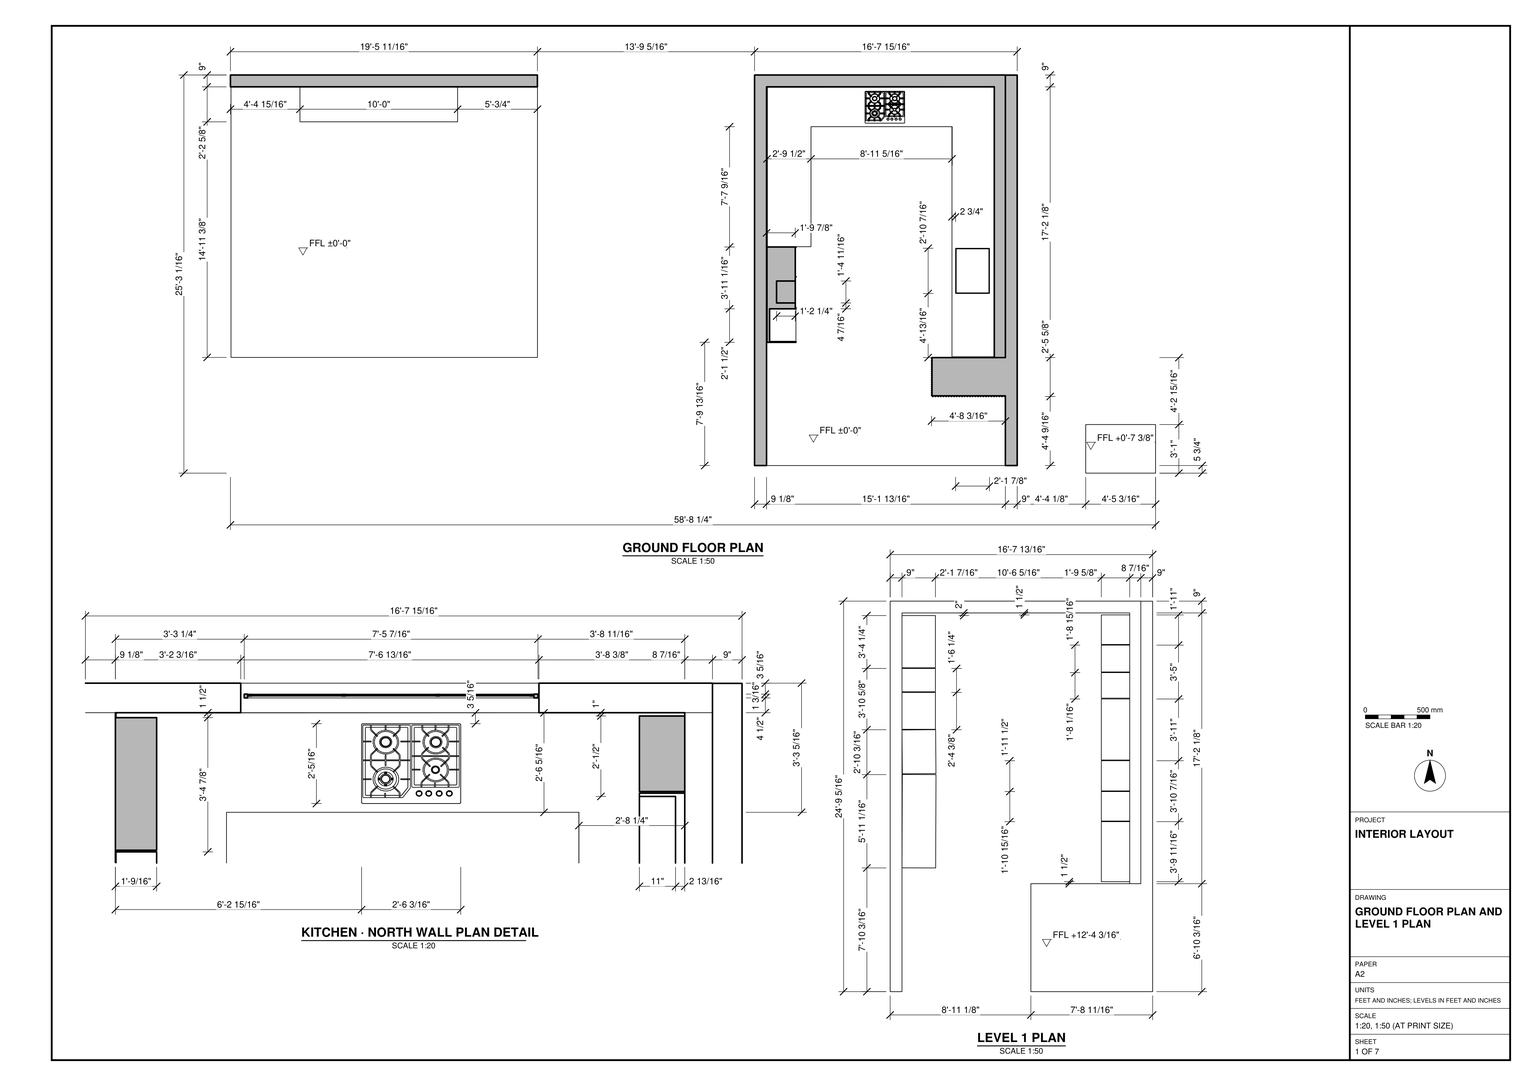
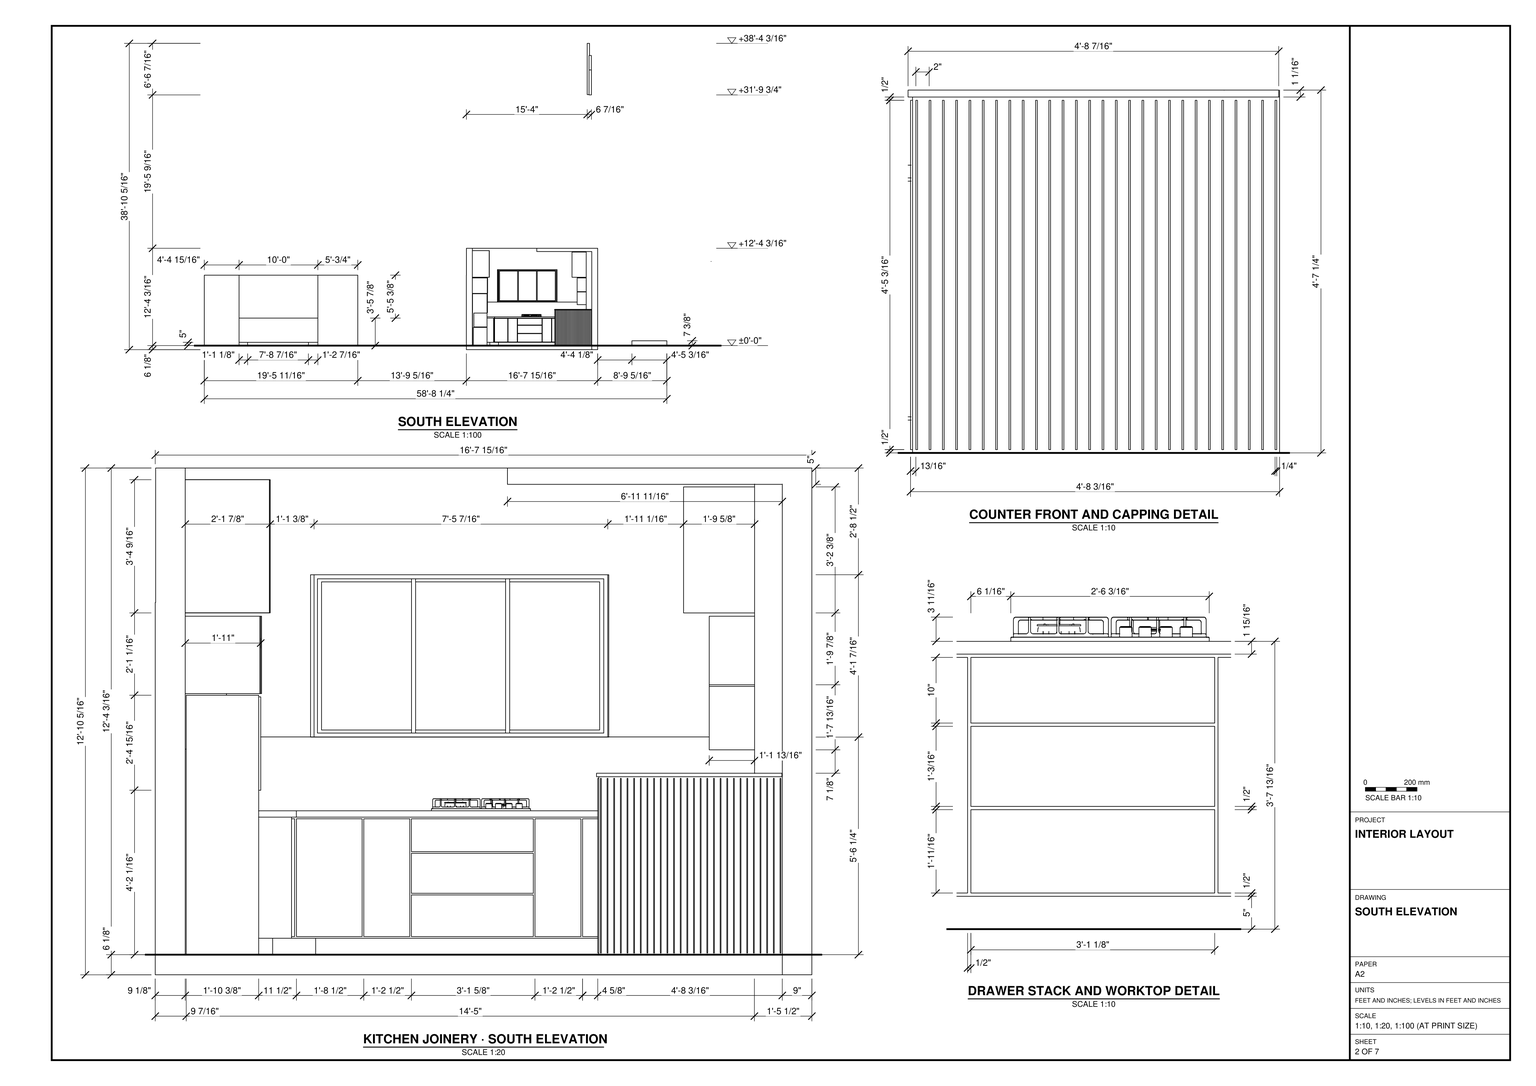
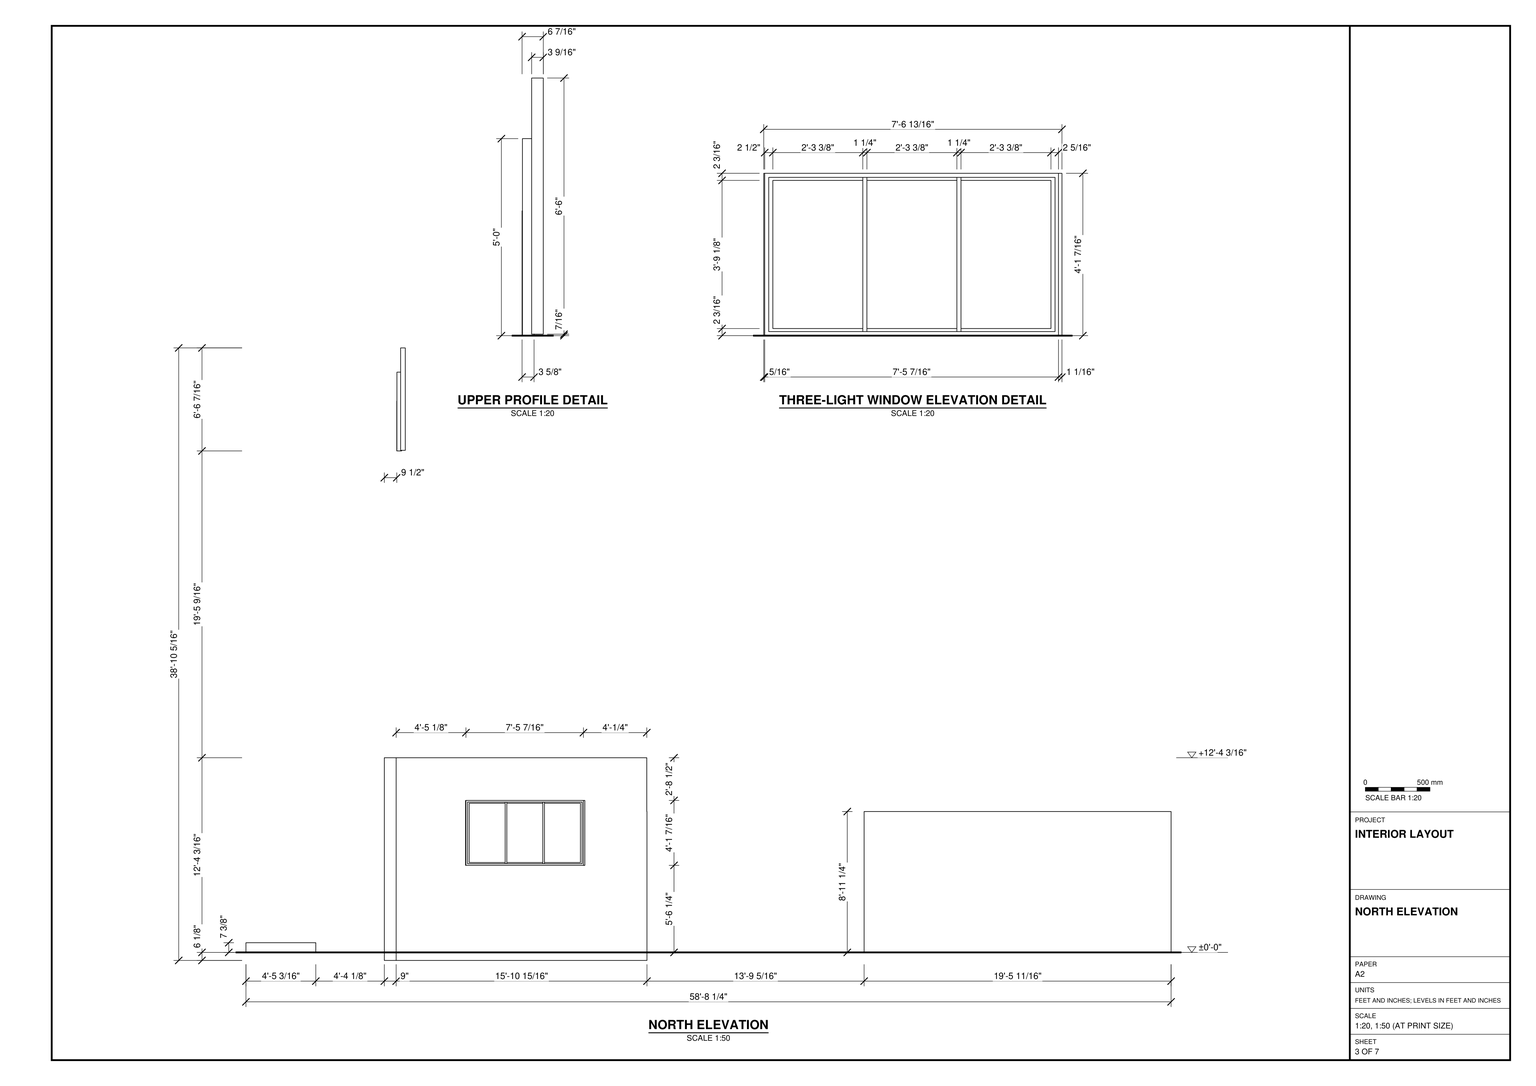
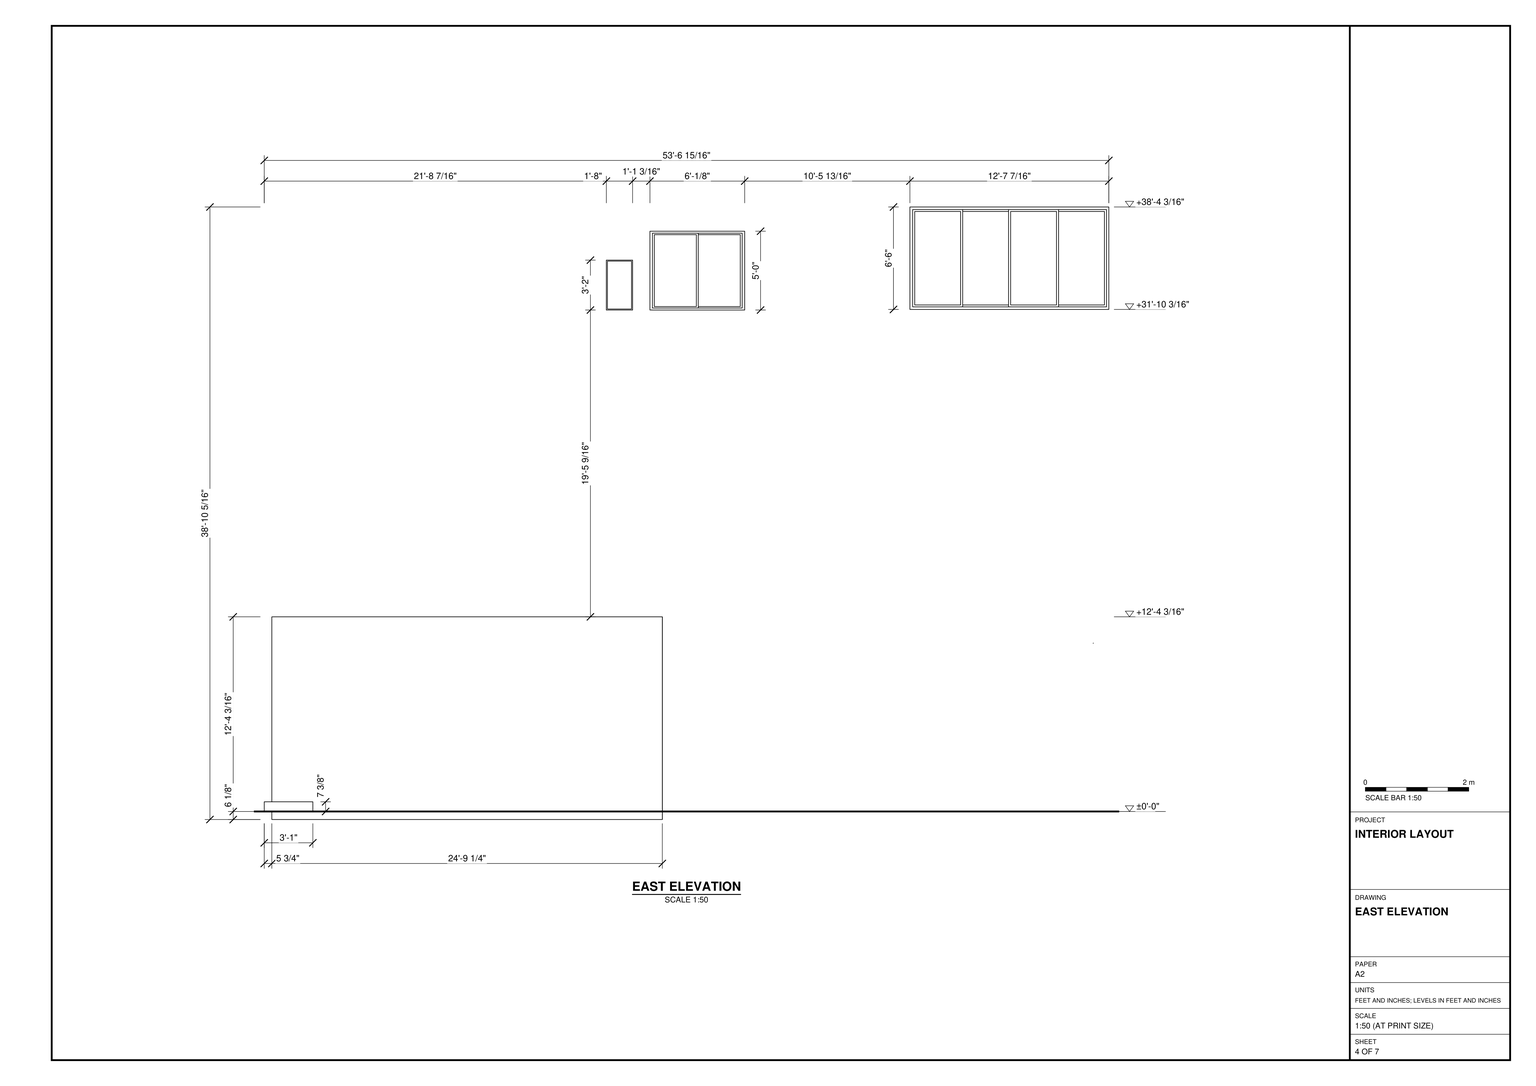
Build the interior layout in SketchUp from task_files/diagram_01.pdf. Work in feet and inches. The overall model extents are 58'-8 1/4" east to west, 53'-6 15/16" north to south and 38'-10 5/16" vertically. Use ±0'-0" as the ground-floor datum and +12'-4 3/16" as the Level 1 datum.

Set out the kitchen floor slab and its three enclosing walls, using the wall thicknesses shown in plan and leaving the south side open as drawn. Fit the framed three-light window into the north wall. Use the joinery plans and elevations together to lay out the side runs, storage divisions and worktops. Place the drawer stack beneath the cooktop on the north run. At the south end of the east run, model the projecting counter with its vertically ribbed front and thin cap.

Reproduce the separate wall and projecting unit west of the kitchen, the low rectangular block to the east and the stepped upper profile at the height shown in elevation. Preserve the gaps between these elements. Keep each shell element and each piece of furniture or joinery in a separate group or component, and use components for repeated parts. Decor, loose items and appliances may be any suitable library components. Save one SketchUp model as output_files/kitchen_interior_and_surrounding_layout.skp.

# SketchUp Ruby script. Lengths in inches.
U = 1.inch
M = Sketchup.active_model
def pt(a) = Geom::Point3d.new(a.map { |v| v * U })
def face(e, loops, mat)
  f = e.add_face(loops[0].map { |a| pt(a) })
  loops[1..].each { |l| e.add_face(l.map { |a| pt(a) }).erase! }
  f.material = f.back_material = mat if mat
  f
end
# faces: each face lists its corners as indices into pts; further lists are holes
def faces(e, pts, list, mat = nil) = list.each { |f| face(e, (f[0].is_a?(Array) ? f : [f]).map { |l| l.map { |i| pts[i] } }, mat) }
# xy, xz, yz: faces in a plane at the given z, y or x. An outline is a flat list of corners, or four numbers for a rectangle; further outlines are holes
def ring(l) = l.size == 4 ? [[l[0], l[1]], [l[2], l[1]], [l[2], l[3]], [l[0], l[3]]] : l.each_slice(2).to_a
def flat(e, list, mat, &to3) = list.each { |f| face(e, (f[0].is_a?(Array) ? f : [f]).map { |l| ring(l).map { |u, v| to3.(u, v) } }, mat) }
def xy(e, z, list, mat = nil) = flat(e, list, mat) { |x, y| [x, y, z] }
def xz(e, y, list, mat = nil) = flat(e, list, mat) { |x, z| [x, y, z] }
def yz(e, x, list, mat = nil) = flat(e, list, mat) { |y, z| [x, y, z] }
def lines(e, pts, list) = list.each { |a, b| e.add_line(pt(pts[a]), pt(pts[b])) }
# prism: a flat outline (further loops are holes) pulled along v
def prism(e, loops, v, mat = nil)
  f = face(e, loops, mat); d = Geom::Vector3d.new(v.map { |x| x * U })
  f.pushpull(f.normal.samedirection?(d) ? d.length : -d.length)
end
def box(e, o, s, mat = nil) = prism(e, [[o, [o[0] + s[0], o[1], o[2]], [o[0] + s[0], o[1] + s[1], o[2]], [o[0], o[1] + s[1], o[2]]]], [0, 0, s[2]], mat)
def at(x, y, z, deg = 0) = Geom::Transformation.translation(pt([x, y, z])) * Geom::Transformation.rotation(ORIGIN, Z_AXIS, deg.degrees)
def axes(o, x, y, z) = Geom::Transformation.new([*x, 0, *y, 0, *z, 0, *pt(o).to_a, 1])
def part(name) = M.definitions.add(name)
# library, detail: a bought-in or finely detailed component or shape, given as its bounding box
def library(name, o, s) = part(name).tap { |d| box(d.entities, o, s) }
def detail(e, o, s) = box(e.add_group.entities, o, s)
def put(e, d, t, mat = nil) = e.add_instance(d, t).tap { |i| i.material = mat if mat }
def group(e, t, mat = nil) = e.add_group.tap { |g| g.transformation = t; g.material = mat if mat }.entities
root = M.entities
M.materials.add("Glass Clear 001").color = [0, 0, 0]
M.materials["Glass Clear 001"].alpha = 0.1
M.materials.add("Marble White 23-64 150cm").color = [203, 197, 196]
M.materials.add("Tiles White 03 60cm").color = [173, 178, 172]
M.materials.add("[0010_Snow]").color = [255, 250, 250]
M.materials.add("[0031_PapayaWhip]").color = [255, 239, 213]
M.materials.add("[0095_LightBlue]").color = [173, 216, 230]
M.materials.add("[0135_DarkGray]").color = [81, 81, 81]
M.materials.add("[Carrera Marble]").color = [207, 207, 207]
M.materials.add("[Metal Aluminum Anodized]").color = [202, 209, 219]
M.materials.add("[Metal Seamed]").color = [118, 119, 115]
M.materials.add("[Translucent Glass Tinted]").color = [1, 25, 30]
M.materials["[Translucent Glass Tinted]"].alpha = 0.31
c1 = part("Group\#98")
g1 = group(c1.entities,at(-0.375,0,0),"[Metal Seamed]")
prism(g1,[[[0.375,0,0],[0.375,0,57],[0.375,26.94,57],[0.375,26.94,0]],[[0.375,25.82,55.875],[0.375,1.125,55.875],[0.375,1.125,1.125],[0.375,25.82,1.125]]],[1.5,0,0])
g2 = group(c1.entities,at(0.18,24.32,1.125),"[Translucent Glass Tinted]")
box(g2,[0,-23.19,0],[1.125,24.69,54.75])
c2 = part("Group\#74")
prism(c2.entities,[[[0,0,60],[0,56.89,60],[0,56.89,0],[0,0,0]],[[0,0.78,1.5],[0,56.23,1.5],[0,56.23,58.5],[0,0.78,58.5]]],[3.6875,0,0])
c3 = part("Aluminium+Channel+Glass+Window")
put(c3.entities,c1,axes([-81.68,-37.83,338.57],[2.53703,0,0],[0,0.7423,0],[0,0,0.66667]))
g3 = group(c3.entities,at(-184.95,0.34,23.07))
put(g3,c1,axes([-8.69,0.59,1.24],[0,0.31546,0],[-1.15548,0,0],[0,0,0.82396]))
put(g3,c2,axes([52.25,0,0],[0,0.31546,0],[-1.63756,0,0],[0,0,0.82396]),"[Metal Aluminum Anodized]")
put(g3,c1,axes([50.97,0.59,1.24],[0,0.31546,0],[-1.15548,0,0],[0,0,0.82396]))
put(g3,c1,axes([21.14,0.59,1.24],[0,0.31546,0],[-1.15548,0,0],[0,0,0.82396]))
g4 = group(c3.entities,at(-84.6,278.21,339.02))
put(g4,c1,axes([1.875,-9.85,1.95],[1,0,0],[0,1.41373,0],[0,0,1.3]))
put(g4,c2,axes([0,-84.93,0],[1,0,0],[0,2.66186,0],[0,0,1.3]),"[Metal Aluminum Anodized]")
put(g4,c1,axes([0.375,26.65,1.95],[1,0,0],[0,1.41373,0],[0,0,1.3]))
put(g4,c1,axes([1.875,-82.85,1.95],[1,0,0],[0,1.41373,0],[0,0,1.3]))
put(g4,c1,axes([0.375,-46.35,1.95],[1,0,0],[0,1.41373,0],[0,0,1.3]))
g5 = group(c3.entities,at(-81.68,-4.64,338.57))
g6 = group(g5,at(0,0,0),"[Metal Aluminum Anodized]")
prism(g6,[[[0,0,60],[0,72.13,60],[0,72.13,0],[0,0,0]],[[0,1.9,1.5],[0,70.23,1.5],[0,70.23,58.5],[0,1.9,58.5]]],[3.6875,0,0])
put(g5,c1,axes([1.875,1.9,1.5],[1,0,0],[0,1.29496,0],[0,0,1]))
put(g5,c1,axes([0.375,35.34,1.5],[1,0,0],[0,1.29496,0],[0,0,1]))
c4 = library("Группа\#68",[0,0,-0.08],[23.6,20.47,1.99])
c5 = part("варочная+панель")
p = [[285.71,355.65,85.04],[285.71,355.46,84.84]]
lines(c5.entities,p,[[0,1]])
put(c5.entities,c3,at(173.85,22.72,0))
put(c5.entities,c4,axes([-14.79,-9.1,0.78],[1.3328,0,0],[0,1.188,0],[0,0,1.86]))
c6 = library("Group\#5",[-0.3125,-0.5,0],[56.1875,29.625,54.18])
box(root,[651.09,0,0],[53.19,37,7.375],"[0135_DarkGray]")
xy(root,-6.125,[[399,5.78,589.9375,303.09]],"[0031_PapayaWhip]")
xy(root,-6.125,[[589.9375,5.78,598.9375,303.03]],"[0095_LightBlue]")
xy(root,0,[[[399,5.78,589.9375,5.78,589.9375,58.84,534.0625,58.84,534.0625,87.97,589.9375,87.97,589.9375,303.09,399,303.09],[408.4375,99.59,408.4375,172.17,430.5,172.17,430.5,171.79,430,171.79,430,149.7,430.5,149.7,430.5,149.31,430,149.31,430,125.97,430.5,125.97,430.5,99.59]]],"Marble White 23-64 150cm")
xy(root,0,[[534.0625,58.84,589.9375,87.97],[0.4375,88.09,233.75,88.09,233.75,294.09,172.9375,294.09,172.9375,277.92,52.9375,277.92,52.9375,294.09,0.4375,294.09]],"[0135_DarkGray]")
xy(root,0.5,[[409.6875,100.09,430.5,125.09]],"[0135_DarkGray]")
xy(root,2,[[415.75,129.55,430,146.26]],"[0135_DarkGray]")
xy(root,5.5,[[549.72,132.17,550.625,159.02],[442,266.64,462,267.45],[462.5,266.64,476.5,267.45],[477,266.64,514.125,267.45],[514.625,266.64,528.625,267.45],
  [529.125,266.64,549.125,267.45]],"[0135_DarkGray]")
xy(root,18.1875,[[477,266.64,514.125,267.45]],"[0095_LightBlue]")
xy(root,18.6875,[[477,266.64,514.125,267.45]],"[0135_DarkGray]")
xy(root,19.9375,[[415.75,129.55,430,146.26]],"[0135_DarkGray]")
xy(root,22.3125,[[415.75,129.55,430,146.26]],"[0135_DarkGray]")
xy(root,27.75,[[409.6875,100.09,430.5,125.09]],"[0135_DarkGray]")
xy(root,28.4375,[[410.4375,100.09,430.5,125.09]],"[0135_DarkGray]")
xy(root,30.875,[[477,266.64,514.125,267.45]],"[0095_LightBlue]")
xy(root,31.375,[[477,266.64,514.125,267.45]],"[0135_DarkGray]")
xy(root,34.375,[[415.75,129.55,430,146.26]],"[0135_DarkGray]")
xy(root,36,[[415.75,129.55,430,146.26]],"[0135_DarkGray]")
xy(root,41.375,[[442,266.64,462,267.45],[477,266.64,514.125,267.45],[514.625,266.64,528.625,267.45],[529.125,266.64,549.125,267.45]],"[0095_LightBlue]")
xy(root,41.375,[[549.72,132.17,550.625,159.02],[462.5,266.64,476.5,267.45]],"[0135_DarkGray]")
xy(root,41.875,[[[549.28,88.58,549.28,263.75,441.96,263.75,441.96,172.39,408.4375,172.39,408.4375,294.09,581.5,294.09,581.5,88.58],[552.53,137.27,577.375,170.7]]],"[0135_DarkGray]")
xy(root,43.125,[[[552.03,136.77,577.875,171.2],[552.53,137.27,577.375,170.7]]],"[0135_DarkGray]")
xy(root,43.8125,[[[549.28,88.58,581.5,88.58,581.5,294.09,408.4375,294.09,408.4375,172.39,441.96,172.39,441.96,263.75,549.28,263.75],[552.03,136.77,577.875,171.2]]],"[Carrera Marble]")
xy(root,48.625,[[415.75,129.55,430,146.26]],"[0135_DarkGray]")
xy(root,49.5625,[[410.4375,100.09,430.5,125.09]],"[0135_DarkGray]")
xy(root,50.0625,[[430.5,100.09,431.125,125.09]],"[0135_DarkGray]")
xy(root,50.8125,[[415.75,129.55,430,146.26]],"[0135_DarkGray]")
xy(root,54.18,[[533.375,56.78,589.8125,88.03]],"Marble White 23-64 150cm")
xy(root,55.25,[[533.375,56.78,589.8125,88.03]],"[Carrera Marble]")
xy(root,62.375,[[567.6875,89.47,581.5,113.97],[567.6875,114.47,581.5,158.09],[567.6875,158.59,581.5,181.59],[567.6875,182.09,581.5,205.09],[567.6875,205.59,581.5,228.59],
  [567.6875,229.09,581.5,269.59],[567.6875,270.09,581.5,293.09]],"[0095_LightBlue]")
xy(root,62.59,[[408.125,172.17,420.6875,205.22],[408.125,205.72,420.6875,233.97],[408.125,234.47,420.6875,251.72],[408.125,252.22,420.6875,292.59]],"[0095_LightBlue]")
xy(root,63.25,[[415.75,129.55,430,146.26]],"[0135_DarkGray]")
xy(root,63.375,[[567.6875,90.47,578.4375,112.97],[567.6875,115.47,581.5625,157.09],[567.6875,183.09,580.9375,204.09],[567.6875,230.09,578.375,268.59]],"[0095_LightBlue]")
xy(root,65.8125,[[415.75,129.55,430,146.26]],"[0135_DarkGray]")
xy(root,71.02,[[567.6875,230.09,578.375,268.59]],"[0095_LightBlue]")
xy(root,71.61,[[567.6875,230.09,578.375,268.59]],"[0095_LightBlue]")
xy(root,71.64,[[567.6875,115.47,581.5,157.09]],"[0095_LightBlue]")
xy(root,72.24,[[567.6875,115.47,581.5,157.09]],"[0095_LightBlue]")
xy(root,77.25,[[415.75,129.55,430,146.26]],"[0135_DarkGray]")
xy(root,78.5,[[430.5,100.09,431.125,125.09],[430,125.97,430.5,129.55],[430,129.55,430.5,146.26],[430,146.26,430.5,146.54],[430,146.54,430.5,149.31],
  [430,149.7,430.5,171.79]],"[0135_DarkGray]")
xy(root,79,[[408.4375,99.59,430.5,100.09],[408.4375,100.09,430.5,125.09],[408.4375,125.09,430.5,125.59],[408.4375,125.59,430.5,149.31],[408.4375,149.31,430.5,149.7],
  [408.4375,149.7,430.5,171.67],[408.4375,171.67,430.5,172.17]],"[0135_DarkGray]")
xy(root,79.5,[[430.85,99.39,408.125,99.55,408.38,137.43,431.11,137.28],[431.12,137.75,408.125,137.92,408.38,171.61,431.375,171.4375]],"[0135_DarkGray]")
xy(root,80.6875,[[567.6875,90.47,578.4375,112.97],[567.6875,115.47,581.5625,157.09],[567.6875,183.09,580.9375,204.09],[567.6875,230.09,578.375,268.59]],"[0095_LightBlue]")
xy(root,81.6875,[[567.6875,89.47,581.5,113.97],[567.6875,114.47,581.5,158.09],[567.6875,182.09,581.5,205.09],[567.6875,229.09,581.5,269.59]],"[0135_DarkGray]")
xy(root,82.1875,[[567.6875,89.47,581.5,113.97],[567.6875,114.47,581.5,158.09],[567.6875,182.09,581.5,205.09],[567.6875,229.09,581.5,269.59]],"[0135_DarkGray]")
xy(root,83.1875,[[567.6875,90.47,580.3125,112.97],[567.6875,115.47,581.5,157.09],[567.6875,183.09,581,204.09],[567.6875,230.09,578.6875,268.59]],"[0095_LightBlue]")
xy(root,91.1875,[[567.6875,115.47,581.5,157.09]],"[0095_LightBlue]")
xy(root,91.33,[[567.6875,230.09,578.6875,268.59]],"[0135_DarkGray]")
xy(root,91.8,[[567.6875,115.47,581.5,157.09]],"[0095_LightBlue]")
xy(root,91.92,[[567.6875,230.09,578.6875,268.59]],"[0095_LightBlue]")
xy(root,102.0625,[[567.6875,90.47,580.3125,112.97],[567.6875,115.47,581.5,157.09],[567.6875,183.09,581,204.09],[567.6875,230.09,578.6875,268.59]],"[0095_LightBlue]")
xy(root,103.0625,[[430.85,99.39,431.11,137.28,408.38,137.43,408.125,99.55]],"[0095_LightBlue]")
xy(root,103.0625,[[567.6875,89.47,581.5,113.97],[567.6875,114.47,581.5,158.09],[431.12,137.75,431.375,171.4375,408.38,171.61,408.125,137.92],[567.6875,158.59,581.5,181.59],[408.125,172.17,420.6875,205.22],
  [567.6875,182.09,581.5,205.09],[567.6875,205.59,581.5,228.59],[408.125,205.72,420.6875,233.97],[567.6875,229.09,581.5,269.59],[408.125,234.47,420.6875,251.72],
  [408.125,252.22,420.6875,292.59],[567.6875,270.09,581.5,293.09]],"[0135_DarkGray]")
xy(root,104.0625,[[559.875,89.46,581.5,135.18],[559.875,135.68,581.5,158.12],[559.875,158.62,581.5,181.59],[408.38,171.61,408.125,205.01,433.71,205.21,433.97,171.8125],[559.875,182.12,581.5,228.59],
  [408.125,205.51,433.5625,233.57],[559.875,229.22,581.5,248.65],[408.125,234.07,433.5625,251.82],[559.875,249.15,581.5,269.59],[408.125,252.32,433.5625,292.09],
  [559.875,270.09,581.5,292.59]],"[0095_LightBlue]")
xy(root,104.11,[[433.75,99.96,408.125,100.05,408.38,171.11,434.01,171.02]],"[0095_LightBlue]")
xy(root,142.4375,[[559.875,89.46,581.5,135.18],[559.875,135.68,581.5,158.12],[559.875,158.62,581.5,181.59],[559.875,182.12,581.5,228.59],[559.875,229.22,581.5,248.65],
  [559.875,249.15,581.5,269.59],[559.875,270.09,581.5,292.59]],"[0095_LightBlue]")
xy(root,143.22,[[506.25,5.78,589.9375,87.97]],"[0135_DarkGray]")
xy(root,144.625,[[433.75,99.96,434.01,171.02,408.38,171.11,408.125,100.05],[408.125,205.51,433.5625,233.57],[408.125,234.07,433.5625,251.82],[408.125,252.32,433.5625,292.09]],"[0095_LightBlue]")
xy(root,144.67,[[408.38,171.61,433.97,171.8125,433.71,205.21,408.125,205.01]],"[0095_LightBlue]")
xy(root,148.1875,[[506.25,5.78,598.9375,5.78,598.9375,303.03,589.9375,303.03,589.9375,87.97,506.25,87.97]],"[0135_DarkGray]")
xz(root,5.78,[[399,-6.125,589.9375,0]],"Marble White 23-64 150cm")
xz(root,5.78,[[589.9375,-6.125,598.9375,-6.125,598.9375,148.1875,506.25,148.1875,506.25,143.22,589.9375,143.22]],"[0010_Snow]")
xz(root,56.78,[[533.375,54.18,589.8125,55.25]],"Marble White 23-64 150cm")
xz(root,87.97,[[506.25,143.22,589.9375,148.1875]],"[0135_DarkGray]")
xz(root,88.03,[[533.375,54.18,589.8125,55.25]],"Marble White 23-64 150cm")
xz(root,88.58,[[549.28,41.875,581.5,43.8125]],"[0135_DarkGray]")
xz(root,89.46,[[559.875,104.0625,581.5,142.4375]],"[0095_LightBlue]")
xz(root,89.47,[[567.6875,62.375,581.5,81.6875],[567.6875,82.1875,581.5,103.0625]],"[0135_DarkGray]")
xz(root,90.47,[[567.6875,63.375,578.4375,80.6875],[567.6875,83.1875,580.3125,102.0625]],"[0095_LightBlue]")
xz(root,99.59,[[408.4375,0,430.5,79]],"[0095_LightBlue]")
xz(root,100.09,[[409.6875,0.5,430.5,27.75],[410.4375,28.4375,430.5,49.5625],[430.5,50.0625,431.125,78.5]],"[0135_DarkGray]")
xz(root,112.97,[[567.6875,63.375,578.4375,80.6875],[567.6875,83.1875,580.3125,102.0625]],"[0095_LightBlue]")
xz(root,113.97,[[567.6875,62.375,581.5,81.6875],[567.6875,82.1875,581.5,103.0625]],"[0135_DarkGray]")
xz(root,114.47,[[567.6875,62.375,581.5,81.6875],[567.6875,82.1875,581.5,103.0625]],"[0135_DarkGray]")
xz(root,115.47,[[567.6875,63.375,567.6875,71.64,581.5,71.64,581.5,72.24,567.6875,72.24,567.6875,80.6875,581.5625,80.6875,581.5625,63.375],[567.6875,83.1875,581.5,91.1875],[567.6875,91.8,581.5,102.0625]],"[0095_LightBlue]")
xz(root,115.47,[[567.6875,71.64,581.5,72.24],[567.6875,91.1875,581.5,91.8]],"[0135_DarkGray]")
xz(root,125.09,[[409.6875,0.5,430.5,27.75],[410.4375,28.4375,430.5,49.5625],[430.5,50.0625,431.125,78.5]],"[0135_DarkGray]")
xz(root,125.97,[[430,0,430.5,0.5],[430,0.5,430.5,1.31],[430,1.31,430.5,19.32],[430,19.32,430.5,20.5],[430,20.5,430.5,21],
  [430,21,430.5,21.51],[430,21.51,430.5,34.0625],[430,34.0625,430.5,35],[430,35,430.5,35.5],[430,35.5,430.5,48.125],
  [430,48.125,430.5,49.5],[430,49.5,430.5,50],[430,50,430.5,63.29],[430,63.29,430.5,64],[430,64,430.5,64.5],
  [430,64.5,430.5,66.23],[430,66.23,430.5,78.5]],"[0135_DarkGray]")
xz(root,129.55,[[415.75,2,430,19.9375],[415.75,22.3125,430,34.375],[415.75,36,430,48.625],[415.75,50.8125,430,63.25],[415.75,65.8125,430,77.25]],"[0135_DarkGray]")
xz(root,132.17,[[549.72,5.5,550.625,41.375]],"[0135_DarkGray]")
xz(root,135.18,[[559.875,104.0625,581.5,142.4375]],"[0135_DarkGray]")
xz(root,135.68,[[559.875,104.0625,581.5,142.4375]],"[0135_DarkGray]")
xz(root,136.77,[[552.03,43.125,577.875,43.8125]],"[0135_DarkGray]")
xz(root,137.27,[[552.53,41.875,577.375,43.125]],"[0135_DarkGray]")
xz(root,146.26,[[415.75,2,430,19.9375],[415.75,22.3125,430,34.375],[415.75,36,430,48.625],[415.75,50.8125,430,63.25],[415.75,65.8125,430,77.25]],"[0135_DarkGray]")
xz(root,149.31,[[430,0,430.5,0.5],[430,0.5,430.5,1.71],[430,1.71,430.5,19.25],[430,19.25,430.5,20.5],[430,20.5,430.5,21],
  [430,21,430.5,21.875],[430,21.875,430.5,33.9],[430,33.9,430.5,35],[430,35,430.5,35.5],[430,35.5,430.5,36.53],
  [430,36.53,430.5,49.5],[430,49.5,430.5,50],[430,50,430.5,64],[430,64,430.5,64.5],[430,64.5,430.5,65.16],
  [430,65.16,430.5,78.5]],"[0135_DarkGray]")
xz(root,149.7,[[430,0,430.5,0.5],[430,0.5,430.5,78.5]],"[0135_DarkGray]")
xz(root,157.09,[[567.6875,63.375,581.5625,63.375,581.5625,80.6875,567.6875,80.6875,567.6875,72.24,581.5,72.24,581.5,71.64,567.6875,71.64],[567.6875,83.1875,581.5,91.1875],[567.6875,91.8,581.5,102.0625]],"[0095_LightBlue]")
xz(root,157.09,[[567.6875,71.64,581.5,72.24]],"[0135_DarkGray]")
xz(root,158.09,[[567.6875,62.375,581.5,81.6875],[567.6875,82.1875,581.5,103.0625]],"[0135_DarkGray]")
xz(root,158.12,[[559.875,104.0625,581.5,142.4375]],"[0135_DarkGray]")
xz(root,158.59,[[567.6875,62.375,581.5,103.0625]],"[0135_DarkGray]")
xz(root,158.62,[[559.875,104.0625,581.5,142.4375]],"[0135_DarkGray]")
xz(root,159.02,[[549.72,5.5,550.625,41.375]],"[0135_DarkGray]")
xz(root,170.7,[[552.53,41.875,577.375,43.125]],"[0135_DarkGray]")
xz(root,171.2,[[552.03,43.125,577.875,43.8125]],"[0135_DarkGray]")
xz(root,171.79,[[430,0,430.5,0.5],[430,0.5,430.5,78.5]],"[0135_DarkGray]")
xz(root,172.17,[[408.4375,0,408.4375,62.59,420.6875,62.59,420.6875,79,430.5,79,430.5,0]],"[0095_LightBlue]")
xz(root,172.17,[[408.125,62.59,408.4375,62.59,408.4375,79,420.6875,79,420.6875,103.0625,408.125,103.0625],[408.4375,62.59,420.6875,79]],"[0135_DarkGray]")
xz(root,172.39,[[408.4375,41.875,441.96,43.8125]],"[Carrera Marble]")
xz(root,181.59,[[567.6875,62.375,581.5,103.0625],[559.875,104.0625,581.5,142.4375]],"[0135_DarkGray]")
xz(root,182.09,[[567.6875,62.375,581.5,81.6875],[567.6875,82.1875,581.5,103.0625]],"[0135_DarkGray]")
xz(root,182.12,[[559.875,104.0625,581.5,142.4375]],"[0135_DarkGray]")
xz(root,183.09,[[567.6875,63.375,580.9375,80.6875],[567.6875,83.1875,581,102.0625]],"[0095_LightBlue]")
xz(root,204.09,[[567.6875,63.375,580.9375,80.6875],[567.6875,83.1875,581,102.0625]],"[0095_LightBlue]")
xz(root,205.09,[[567.6875,62.375,581.5,81.6875],[567.6875,82.1875,581.5,103.0625]],"[0135_DarkGray]")
xz(root,205.22,[[408.125,62.59,420.6875,103.0625]],"[0135_DarkGray]")
xz(root,205.51,[[408.125,104.0625,433.5625,144.625]],"[0135_DarkGray]")
xz(root,205.59,[[567.6875,62.375,581.5,103.0625]],"[0135_DarkGray]")
xz(root,205.72,[[408.125,62.59,420.6875,103.0625]],"[0135_DarkGray]")
xz(root,228.59,[[567.6875,62.375,581.5,103.0625],[559.875,104.0625,581.5,142.4375]],"[0135_DarkGray]")
xz(root,229.09,[[567.6875,62.375,581.5,81.6875],[567.6875,82.1875,581.5,103.0625]],"[0135_DarkGray]")
xz(root,229.22,[[559.875,104.0625,581.5,142.4375]],"[0135_DarkGray]")
xz(root,230.09,[[567.6875,63.375,578.375,71.02],[567.6875,71.61,578.375,80.6875],[567.6875,83.1875,578.6875,91.33],[567.6875,91.92,578.6875,102.0625]],"[0095_LightBlue]")
xz(root,230.09,[[567.6875,71.02,578.375,71.61],[567.6875,91.33,578.6875,91.92]],"[0135_DarkGray]")
xz(root,233.57,[[408.125,104.0625,433.5625,144.625]],"[0135_DarkGray]")
xz(root,233.97,[[408.125,62.59,420.6875,103.0625]],"[0135_DarkGray]")
xz(root,234.07,[[408.125,104.0625,433.5625,144.625]],"[0135_DarkGray]")
xz(root,234.47,[[408.125,62.59,420.6875,103.0625]],"[0135_DarkGray]")
xz(root,248.65,[[559.875,104.0625,581.5,142.4375]],"[0135_DarkGray]")
xz(root,249.15,[[559.875,104.0625,581.5,142.4375]],"[0135_DarkGray]")
xz(root,251.72,[[408.125,62.59,420.6875,103.0625]],"[0135_DarkGray]")
xz(root,251.82,[[408.125,104.0625,433.5625,144.625]],"[0135_DarkGray]")
xz(root,252.22,[[408.125,62.59,420.6875,103.0625]],"[0135_DarkGray]")
xz(root,252.32,[[408.125,104.0625,433.5625,144.625]],"[0135_DarkGray]")
xz(root,263.75,[[441.96,41.875,549.28,43.8125]],"[Carrera Marble]")
xz(root,266.64,[[442,5.5,462,41.375],[462.5,5.5,476.5,41.375],[477,5.5,514.125,18.1875],[514.625,5.5,528.625,41.375],[529.125,5.5,549.125,41.375],
  [477,18.6875,514.125,30.875],[477,31.375,514.125,41.375]],"[0095_LightBlue]")
xz(root,267.45,[[442,5.5,462,41.375],[462.5,5.5,476.5,41.375],[477,5.5,514.125,18.1875],[514.625,5.5,528.625,41.375],[529.125,5.5,549.125,41.375],
  [477,18.6875,514.125,30.875],[477,31.375,514.125,41.375]],"[0135_DarkGray]")
xz(root,268.59,[[567.6875,63.375,578.375,71.02],[567.6875,71.61,578.375,80.6875],[567.6875,83.1875,578.6875,91.33],[567.6875,91.92,578.6875,102.0625]],"[0095_LightBlue]")
xz(root,269.59,[[567.6875,62.375,581.5,81.6875],[567.6875,82.1875,581.5,103.0625],[559.875,104.0625,581.5,142.4375]],"[0135_DarkGray]")
xz(root,270.09,[[567.6875,62.375,581.5,103.0625],[559.875,104.0625,581.5,142.4375]],"[0135_DarkGray]")
xz(root,292.09,[[408.125,104.0625,433.5625,144.625]],"[0135_DarkGray]")
xz(root,292.59,[[408.125,62.59,420.6875,103.0625],[559.875,104.0625,581.5,142.4375]],"[0135_DarkGray]")
xz(root,293.09,[[567.6875,62.375,581.5,103.0625]],"[0135_DarkGray]")
xz(root,294.09,[[408.4375,41.875,581.5,43.8125]],"[0135_DarkGray]")
xz(root,303.03,[[589.9375,-6.125,598.9375,148.1875]],"[0135_DarkGray]")
xz(root,303.09,[[399,-6.125,589.9375,0]],"[0135_DarkGray]")
yz(root,399,[[5.78,-6.125,303.09,0]],"[0135_DarkGray]")
yz(root,408.125,[[172.17,62.59,205.22,103.0625],[205.72,62.59,233.97,103.0625],[234.47,62.59,251.72,103.0625],[252.22,62.59,292.59,103.0625],[205.51,104.0625,233.57,144.625],
  [234.07,104.0625,251.82,144.625],[252.32,104.0625,292.09,144.625]],"[0135_DarkGray]")
yz(root,408.4375,[[99.59,0,125.59,79],[125.59,0,172.17,79],[172.17,41.875,172.39,43.8125],[172.39,41.875,294.09,43.8125]],"[0135_DarkGray]")
yz(root,409.6875,[[100.09,0.5,125.09,27.75]],"[0135_DarkGray]")
yz(root,410.4375,[[100.09,28.4375,125.09,49.5625]],"[0135_DarkGray]")
yz(root,415.75,[[129.55,2,146.26,19.9375],[129.55,22.3125,146.26,34.375],[129.55,36,146.26,48.625],[129.55,50.8125,146.26,63.25],[129.55,65.8125,146.26,77.25]],"[0135_DarkGray]")
yz(root,420.6875,[[172.17,62.59,205.22,103.0625],[205.72,62.59,233.97,103.0625],[234.47,62.59,251.72,103.0625],[252.22,62.59,292.59,103.0625]],"[0095_LightBlue]")
yz(root,430,[[129.55,2,146.26,19.9375],[129.55,22.3125,146.26,34.375],[129.55,36,146.26,48.625],[129.55,50.8125,146.26,63.25],[129.55,65.8125,146.26,77.25]],"Glass Clear 001")
yz(root,430,[[149.7,0.5,171.79,78.5]],"[0095_LightBlue]")
yz(root,430,[[125.97,0,149.31,0,149.31,0.5,146.26,0.5,146.26,2,129.55,2,129.55,0.5,125.97,0.5],[149.7,0,171.79,0.5],[125.97,0.5,129.55,20.5],[146.26,0.5,149.31,20.5],[129.55,19.9375,146.26,19.9375,146.26,20.5,149.31,20.5,149.31,21,146.26,21,146.26,22.3125,129.55,22.3125,129.55,21,125.97,21,125.97,20.5,129.55,20.5],
  [125.97,21,129.55,35],[146.26,21,149.31,35],[129.55,34.375,146.26,34.375,146.26,35,149.31,35,149.31,35.5,146.26,35.5,146.26,36,129.55,36,129.55,35.5,125.97,35.5,125.97,35,129.55,35],[125.97,35.5,129.55,49.5],[146.26,35.5,149.31,49.5],
  [129.55,48.625,146.26,48.625,146.26,49.5,149.31,49.5,149.31,50,146.26,50,146.26,50.8125,129.55,50.8125,129.55,50,125.97,50,125.97,49.5,129.55,49.5],[125.97,50,129.55,64],[146.26,50,149.31,64],[129.55,63.25,146.26,63.25,146.26,64,149.31,64,149.31,64.5,146.26,64.5,146.26,65.8125,129.55,65.8125,129.55,64.5,125.97,64.5,125.97,64,129.55,64],[125.97,64.5,129.55,78.5],
  [146.26,64.5,149.31,78.5],[129.55,77.25,146.26,78.5]],"[0135_DarkGray]")
yz(root,430.5,[[[99.59,0,125.59,79],[100.09,50.0625,125.09,78.5],[100.09,0.5,125.09,27.75],[100.09,28.4375,125.09,49.5625]],[125.59,0,125.97,0,125.97,78.5,149.31,78.5,149.31,0,149.7,0,149.7,78.5,171.79,78.5,171.79,0,172.17,0,172.17,79,125.59,79]],"[0135_DarkGray]")
yz(root,431.125,[[100.09,50.0625,125.09,78.5]],"[0095_LightBlue]")
yz(root,433.5625,[[205.51,104.0625,233.57,144.625],[234.07,104.0625,251.82,144.625],[252.32,104.0625,292.09,144.625]],"[0095_LightBlue]")
yz(root,441.96,[[172.39,41.875,263.75,43.8125]],"[Carrera Marble]")
yz(root,442,[[266.64,5.5,267.45,41.375]],"[0135_DarkGray]")
yz(root,462,[[266.64,5.5,267.45,41.375]],"[0095_LightBlue]")
yz(root,462.5,[[266.64,5.5,267.45,41.375]],"[0095_LightBlue]")
yz(root,476.5,[[266.64,5.5,267.45,41.375]],"[0095_LightBlue]")
yz(root,477,[[266.64,5.5,267.45,18.1875],[266.64,18.6875,267.45,30.875],[266.64,31.375,267.45,41.375]],"[0095_LightBlue]")
yz(root,506.25,[[5.78,143.22,87.97,148.1875]],"[0135_DarkGray]")
yz(root,514.125,[[266.64,5.5,267.45,18.1875],[266.64,18.6875,267.45,30.875],[266.64,31.375,267.45,41.375]],"[0095_LightBlue]")
yz(root,514.625,[[266.64,5.5,267.45,41.375]],"[0095_LightBlue]")
yz(root,528.625,[[266.64,5.5,267.45,41.375]],"[0095_LightBlue]")
yz(root,529.125,[[266.64,5.5,267.45,41.375]],"[0095_LightBlue]")
yz(root,533.375,[[56.78,54.18,88.03,55.25]],"Marble White 23-64 150cm")
yz(root,549.125,[[266.64,5.5,267.45,41.375]],"[0135_DarkGray]")
yz(root,549.28,[[88.58,41.875,263.75,43.8125]],"[Carrera Marble]")
yz(root,549.72,[[132.17,5.5,159.02,41.375]],"[0095_LightBlue]")
yz(root,550.625,[[132.17,5.5,159.02,41.375]],"[0135_DarkGray]")
yz(root,552.03,[[136.77,43.125,171.2,43.8125]],"[0135_DarkGray]")
yz(root,552.53,[[137.27,41.875,170.7,43.125]],"[0135_DarkGray]")
yz(root,559.875,[[89.46,104.0625,135.18,142.4375],[135.68,104.0625,158.12,142.4375],[158.62,104.0625,181.59,142.4375],[182.12,104.0625,228.59,142.4375],[229.22,104.0625,248.65,142.4375],
  [249.15,104.0625,269.59,142.4375],[270.09,104.0625,292.59,142.4375]],"[0095_LightBlue]")
yz(root,567.6875,[[90.47,63.375,112.97,80.6875],[115.47,63.375,157.09,71.64],[183.09,63.375,204.09,80.6875],[230.09,63.375,268.59,71.02],[230.09,71.61,268.59,80.6875],
  [115.47,72.24,157.09,80.6875],[90.47,83.1875,112.97,102.0625],[115.47,83.1875,157.09,91.1875],[183.09,83.1875,204.09,102.0625],[230.09,83.1875,268.59,91.33],
  [115.47,91.8,157.09,102.0625],[230.09,91.92,268.59,102.0625]],"Glass Clear 001")
yz(root,567.6875,[[158.59,62.375,181.59,103.0625],[205.59,62.375,228.59,103.0625],[270.09,62.375,293.09,103.0625]],"[0095_LightBlue]")
yz(root,567.6875,[[[89.47,62.375,113.97,81.6875],[90.47,63.375,112.97,80.6875]],[[114.47,62.375,158.09,81.6875],[115.47,63.375,157.09,80.6875]],[[182.09,62.375,205.09,81.6875],[183.09,63.375,204.09,80.6875]],[[229.09,62.375,269.59,81.6875],[230.09,63.375,268.59,80.6875]],[230.09,71.02,268.59,71.61],
  [115.47,71.64,157.09,72.24],[[89.47,82.1875,113.97,103.0625],[90.47,83.1875,112.97,102.0625]],[[114.47,82.1875,158.09,103.0625],[115.47,83.1875,157.09,102.0625]],[[182.09,82.1875,205.09,103.0625],[183.09,83.1875,204.09,102.0625]],[[229.09,82.1875,269.59,103.0625],[230.09,83.1875,268.59,102.0625]],
  [115.47,91.1875,157.09,91.8],[230.09,91.33,268.59,91.92]],"[0135_DarkGray]")
yz(root,577.375,[[137.27,41.875,170.7,43.125]],"[0135_DarkGray]")
yz(root,577.875,[[136.77,43.125,171.2,43.8125]],"[0135_DarkGray]")
yz(root,578.375,[[230.09,63.375,268.59,71.02],[230.09,71.61,268.59,80.6875]],"[0095_LightBlue]")
yz(root,578.4375,[[90.47,63.375,112.97,80.6875]],"[0095_LightBlue]")
yz(root,578.6875,[[230.09,83.1875,268.59,91.33],[230.09,91.92,268.59,102.0625]],"[0095_LightBlue]")
yz(root,580.3125,[[90.47,83.1875,112.97,102.0625]],"[0095_LightBlue]")
yz(root,580.9375,[[183.09,63.375,204.09,80.6875]],"[0095_LightBlue]")
yz(root,581,[[183.09,83.1875,204.09,102.0625]],"[0095_LightBlue]")
yz(root,581.5,[[114.47,62.375,158.09,81.6875]],"[0095_LightBlue]")
yz(root,581.5,[[88.58,41.875,294.09,43.8125],[89.47,62.375,113.97,81.6875],[158.59,62.375,181.59,103.0625],[182.09,62.375,205.09,81.6875],[205.59,62.375,228.59,103.0625],
  [229.09,62.375,269.59,81.6875],[270.09,62.375,293.09,103.0625],[115.47,71.64,157.09,72.24],[89.47,82.1875,113.97,103.0625],[[114.47,82.1875,158.09,103.0625],[115.47,91.8,157.09,102.0625],[115.47,83.1875,157.09,91.1875]],
  [182.09,82.1875,205.09,103.0625],[229.09,82.1875,269.59,103.0625],[89.46,104.0625,114.02,142.4375],[114.02,104.0625,135.18,142.4375],[135.68,104.0625,158.12,142.4375],
  [158.62,104.0625,181.59,142.4375],[182.09,104.0625,182.12,142.4375],[182.12,104.0625,205.12,142.4375],[205.12,104.0625,228.59,142.4375],[229.22,104.0625,248.65,142.4375],
  [249.15,104.0625,269.59,142.4375],[270.09,104.0625,292.59,142.4375]],"[0135_DarkGray]")
yz(root,581.5625,[[115.47,63.375,157.09,80.6875]],"[0135_DarkGray]")
yz(root,589.8125,[[56.78,54.18,88.03,55.25]],"[0135_DarkGray]")
yz(root,589.9375,[[5.78,0,5.78,143.22,87.97,143.22,87.97,148.1875,303.03,148.1875,303.03,0,87.97,0,87.97,54.18,58.84,54.18,58.84,0]],"[0010_Snow]")
yz(root,589.9375,[[5.78,-6.125,58.84,0],[58.84,-6.125,87.97,0],[87.97,-6.125,303.03,0],[303.03,-6.125,303.09,0]],"[0031_PapayaWhip]")
yz(root,598.9375,[[5.78,-6.125,303.03,148.1875]],"[0031_PapayaWhip]")
p = [[408.125,99.55,103.0625],[408.125,99.55,79.5],[430.85,99.39,79.5],[430.85,99.39,103.0625],[431.11,137.28,79.5],[431.11,137.28,103.0625],
  [408.38,137.43,103.0625],[408.38,137.43,79.5],[408.125,137.92,103.0625],[408.125,137.92,79.5],[431.12,137.75,79.5],[431.12,137.75,103.0625],
  [431.375,171.4375,79.5],[431.375,171.4375,103.0625],[408.38,171.61,103.0625],[408.38,171.61,79.5],[408.38,171.11,144.625],[408.38,171.11,104.11],
  [408.125,100.05,104.11],[408.125,100.05,144.625],[433.75,99.96,104.11],[433.75,99.96,144.625],[434.01,171.02,104.11],[434.01,171.02,144.625],
  [408.38,171.61,104.0625],[408.38,171.61,144.67],[408.125,205.01,144.67],[408.125,205.01,104.0625],[433.97,171.8125,104.0625],[433.97,171.8125,144.67],
  [433.71,205.21,104.0625],[433.71,205.21,144.67],[554.75,277.92,0],[434.75,277.92,0],[434.75,294.09,0],[554.75,294.09,0],
  [434.75,277.92,5],[434.75,294.09,5],[554.75,277.92,5],[554.75,294.09,5]]
faces(root,p,[[0,1,2,3],[3,2,4,5],[11,10,12,13],[15,14,13,12],[19,18,20,21],[22,23,21,20],[29,28,30,31]],"[0095_LightBlue]")
faces(root,p,[[1,0,6,7],[7,6,5,4],[8,9,10,11],[9,8,14,15],[16,17,18,19],[17,16,23,22],[24,25,26,27],[25,24,28,29],
  [27,26,31,30]],"[0135_DarkGray]")
lines(root,p,[[32,33],[34,33],[32,35],[36,37],[38,39]])
put(root,c5,axes([497.28,275.53,43.18],[0.9602,0,0],[0,1,0],[0,0,1]))
g7 = group(root,at(43.9375,294.09,0),"[0135_DarkGray]")
xy(g7,107.25,[[-43.9375,0,189.75,9]])
xz(g7,0,[[-43.9375,0,9,107.25],[9,0,129,107.25],[129,0,189.75,107.25]])
xz(g7,9,[[-43.9375,0,189.75,107.25]])
yz(g7,-43.9375,[[0,0,9,107.25]])
yz(g7,189.75,[[0,0,9,107.25]])
g8 = group(root,at(52.9375,277.92,0),"[0135_DarkGray]")
xy(g8,5,[[0,-10.47,120,0]])
xy(g8,41.875,[[0,-10.47,120,16.17]])
xz(g8,-10.47,[[0,5,120,41.875]])
xz(g8,0,[[0,0,13.1,5],[13.1,0,105.5625,5],[105.5625,0,120,5]])
xz(g8,16.17,[[0,0,120,41.875]])
yz(g8,0,[[0,0,0,5,-10.47,5,-10.47,41.875,16.17,41.875,16.17,0]])
yz(g8,120,[[0,0,16.17,0,16.17,41.875,-10.47,41.875,-10.47,5,0,5]])
g9 = group(root,at(434.75,277.92,0),"[0095_LightBlue]")
xy(g9,0,[[120,-189.54,146.6875,16.17],[-26.3125,-104.3125,0,16.17]])
xy(g9,5,[[120,-189.54,146.6875,-189.41],[115.875,-189.41,115.875,-10.47,5.75,-10.47,5.75,-104.34,0,-104.34,0,0,120,0,120,-189.41],[120,-189.41,146.6875,0],[-26.3125,-104.34,0,-104.3125],[-26.3125,-104.3125,0,0]])
xy(g9,5.5,[[114.97,-189.09,115.875,-146.25],[114.97,-118.41,115.875,-76.28],[5.75,-103.72,6.6875,-88.53],[5.75,-88.03,6.6875,-60.78],[114.97,-75.78,115.875,-58.91],
  [5.75,-60.28,6.6875,-46.28],[114.97,-58.41,115.875,-44.03],[5.75,-45.78,6.6875,-11.97],[114.5,-43.53,115.875,-11.97]])
xy(g9,18.25,[[114.97,-75.78,115.875,-58.91],[114.5,-43.53,115.875,-11.97]])
xy(g9,18.75,[[114.97,-75.78,115.875,-58.91],[114.6875,-43.53,115.875,-11.97]])
xy(g9,22.6875,[[5.75,-88.03,6.6875,-60.78],[5.75,-45.78,6.6875,-11.97]],"[0135_DarkGray]")
xy(g9,23.125,[[114.97,-118.41,115.875,-76.28]])
xy(g9,23.1875,[[5.75,-88.03,6.6875,-60.78],[5.75,-45.78,6.6875,-11.97]])
xy(g9,23.625,[[114.97,-118.41,115.875,-76.28]])
xy(g9,27.8125,[[114.97,-189.09,115.875,-146.25]])
xy(g9,28.3125,[[114.97,-189.09,115.875,-146.25]])
xy(g9,30.875,[[5.75,-45.78,6.6875,-11.97]],"[0135_DarkGray]")
xy(g9,30.9375,[[114.97,-75.78,115.875,-58.91],[114.6875,-43.53,115.875,-11.97]])
xy(g9,31.375,[[5.75,-45.78,6.6875,-11.97]])
xy(g9,31.4375,[[114.97,-75.78,115.875,-58.91],[114.9375,-43.53,115.875,-11.97]])
xy(g9,41.375,[[114.97,-189.09,115.875,-146.25],[114.97,-118.41,115.875,-76.28],[114.97,-75.78,115.875,-58.91],[114.97,-58.41,115.875,-44.03],[114.9375,-43.53,115.875,-11.97]])
xy(g9,41.375,[[5.75,-103.72,6.6875,-88.53],[5.75,-88.03,6.6875,-60.78],[5.75,-60.28,6.6875,-46.28],[5.75,-45.78,6.6875,-11.97]],"[0135_DarkGray]")
xy(g9,41.875,[[115.875,-189.41,146.6875,-189.41,146.6875,16.17,-26.3125,16.17,-26.3125,-104.34,5.75,-104.34,5.75,-10.47,115.875,-10.47]])
xz(g9,-189.54,[[120,0,146.6875,5]])
xz(g9,-189.41,[[115.875,5,146.6875,41.875]])
xz(g9,-189.09,[[114.97,5.5,115.875,27.8125],[114.97,28.3125,115.875,41.375]])
xz(g9,-146.25,[[114.97,5.5,115.875,27.8125],[114.97,28.3125,115.875,41.375]])
xz(g9,-118.41,[[114.97,5.5,115.875,23.125],[114.97,23.625,115.875,41.375]])
xz(g9,-104.34,[[-26.3125,5,5.75,41.875]])
xz(g9,-104.3125,[[-26.3125,0,0,5]])
xz(g9,-103.72,[[5.75,5.5,6.6875,41.375]],"[0135_DarkGray]")
xz(g9,-88.53,[[5.75,5.5,6.6875,41.375]],"[0135_DarkGray]")
xz(g9,-88.03,[[5.75,5.5,6.6875,22.6875],[5.75,23.1875,6.6875,41.375]],"[0135_DarkGray]")
xz(g9,-76.28,[[114.97,5.5,115.875,23.125],[114.97,23.625,115.875,41.375]])
xz(g9,-75.78,[[114.97,5.5,115.875,18.25],[114.97,18.75,115.875,30.9375],[114.97,31.4375,115.875,41.375]])
xz(g9,-60.78,[[5.75,5.5,6.6875,22.6875],[5.75,23.1875,6.6875,41.375]],"[0135_DarkGray]")
xz(g9,-60.28,[[5.75,5.5,6.6875,41.375]],"[0135_DarkGray]")
xz(g9,-58.91,[[114.97,5.5,115.875,18.25],[114.97,18.75,115.875,30.9375],[114.97,31.4375,115.875,41.375]])
xz(g9,-58.41,[[114.97,5.5,115.875,41.375]])
xz(g9,-46.28,[[5.75,5.5,6.6875,41.375]],"[0135_DarkGray]")
xz(g9,-45.78,[[5.75,5.5,6.6875,22.6875],[5.75,23.1875,6.6875,30.875],[5.75,31.375,6.6875,41.375]],"[0135_DarkGray]")
xz(g9,-44.03,[[114.97,5.5,115.875,41.375]])
xz(g9,-43.53,[[114.5,5.5,115.875,18.25],[114.6875,18.75,115.875,30.9375],[114.9375,31.4375,115.875,41.375]])
xz(g9,-11.97,[[5.75,5.5,6.6875,22.6875],[114.5,5.5,115.875,18.25],[114.6875,18.75,115.875,30.9375],[5.75,23.1875,6.6875,30.875],[5.75,31.375,6.6875,41.375],
  [114.9375,31.4375,115.875,41.375]])
xz(g9,-10.47,[[5.75,5,115.875,41.875]])
xz(g9,0,[[0,0,13.1,5],[13.1,0,105.5625,5],[105.5625,0,120,5]])
xz(g9,16.17,[[-26.3125,0,146.6875,41.875]])
yz(g9,-26.3125,[[-104.3125,0,16.17,5],[-104.34,5,16.17,41.875]])
yz(g9,0,[[-104.3125,0,0,5]])
yz(g9,5.75,[[[-104.34,5,-10.47,41.875],[-45.78,5.5,-11.97,22.6875],[-103.72,5.5,-88.53,41.375],[-60.28,5.5,-46.28,41.375],[-88.03,23.1875,-60.78,41.375],[-88.03,5.5,-60.78,22.6875],[-45.78,31.375,-11.97,41.375],[-45.78,23.1875,-11.97,30.875]]],"[0135_DarkGray]")
yz(g9,6.6875,[[-103.72,5.5,-88.53,41.375],[-88.03,5.5,-60.78,22.6875],[-60.28,5.5,-46.28,41.375],[-45.78,5.5,-11.97,22.6875],[-88.03,23.1875,-60.78,41.375],
  [-45.78,23.1875,-11.97,30.875],[-45.78,31.375,-11.97,41.375]],"[0095_LightBlue]")
yz(g9,114.5,[[-43.53,5.5,-11.97,18.25]],"[0095_LightBlue]")
yz(g9,114.6875,[[-43.53,18.75,-11.97,30.9375]],"[0095_LightBlue]")
yz(g9,114.9375,[[-43.53,31.4375,-11.97,41.375]],"[0095_LightBlue]")
yz(g9,114.97,[[-189.09,5.5,-146.25,27.8125],[-118.41,5.5,-76.28,23.125],[-75.78,5.5,-58.91,18.25],[-58.41,5.5,-44.03,41.375],[-75.78,18.75,-58.91,30.9375],
  [-118.41,23.625,-76.28,41.375],[-189.09,28.3125,-146.25,41.375],[-75.78,31.4375,-58.91,41.375]],"[0095_LightBlue]")
yz(g9,115.875,[[[-189.41,5,-10.47,41.875],[-189.09,5.5,-146.25,27.8125],[-118.41,23.625,-76.28,41.375],[-118.41,5.5,-76.28,23.125],[-189.09,28.3125,-146.25,41.375],[-58.41,5.5,-44.03,41.375],[-43.53,5.5,-11.97,18.25],[-43.53,18.75,-11.97,30.9375],[-43.53,31.4375,-11.97,41.375],[-75.78,5.5,-58.91,18.25],[-75.78,18.75,-58.91,30.9375],[-75.78,31.4375,-58.91,41.375]]],"[0095_LightBlue]")
yz(g9,120,[[-189.54,0,0,5]])
yz(g9,146.6875,[[-189.54,0,16.17,5],[-189.41,5,16.17,41.875]])
p = [[120,16.17,5],[120,16.25,5]]
lines(g9,p,[[0,1]])
g10 = group(root,at(425.75,294.09,0),"[0010_Snow]")
xy(g10,0,[[-26.75,-288.3125,-17.625,0],[155.75,-206.125,164.1875,0]])
xy(g10,66.25,[[20.54,0,111.35,9]])
xy(g10,107.25,[[-26.75,-288.3125,-26.625,9]])
xy(g10,115.6875,[[20.54,0,111.35,9]])
xy(g10,148.1875,[[-26.625,-288.3125,-17.625,-288.3125,-17.625,0,155.75,0,155.75,-206.125,164.1875,-206.125,164.1875,9,-26.625,9]])
xz(g10,-288.3125,[[-26.75,0,-17.625,0,-17.625,148.1875,-26.625,148.1875,-26.625,107.25,-26.75,107.25]])
xz(g10,-206.125,[[155.75,0,164.1875,148.1875]],"[0095_LightBlue]")
xz(g10,0,[[[-17.625,0,155.75,148.1875],[20.54,66.25,111.35,115.6875]]])
xz(g10,9,[[[-26.75,0,-26.75,107.25,-26.625,107.25,-26.625,148.1875,164.1875,148.1875,164.1875,0],[20.54,66.25,111.35,115.6875]]])
yz(g10,-26.75,[[-288.3125,0,9,107.25]])
yz(g10,-26.625,[[-288.3125,107.25,9,148.1875]])
yz(g10,-17.625,[[-288.3125,0,0,148.1875]])
yz(g10,-17.3125,[[-121.92,43.8125,-0.06,43.8125,-0.06,66.3,-121.92,62.59]],"Tiles White 03 60cm")
yz(g10,20.54,[[0,66.25,9,115.6875]])
yz(g10,111.35,[[0,66.25,9,115.6875]])
yz(g10,155.75,[[-206.125,0,0,43.76]])
yz(g10,155.75,[[-206.125,43.76,0,62.25]],"Tiles White 03 60cm")
yz(g10,155.75,[[-206.125,62.25,0,148.1875]],"[0095_LightBlue]")
yz(g10,164.1875,[[-206.125,0,9,148.1875]])
p = [[-17.3125,-0.06,43.8125],[155.75,0,43.8125],[155.75,0,62.25],[155.75,0,66.3],[-17.3125,-0.06,66.3]]
faces(g10,p,[[0,1,2,3,4]],"Tiles White 03 60cm")
put(root,c6,at(534.0625,58.84,0),"[0135_DarkGray]")
